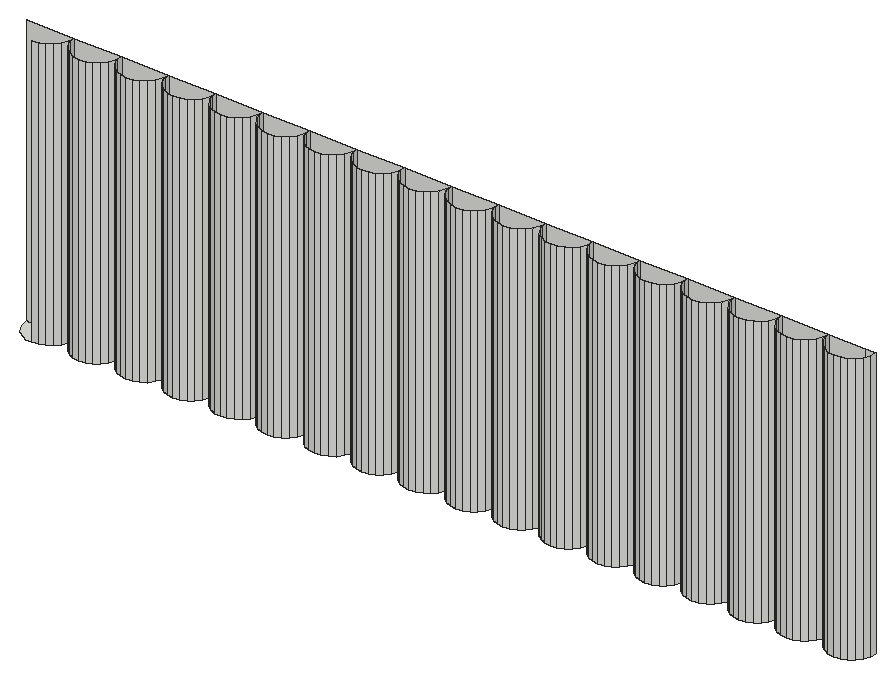
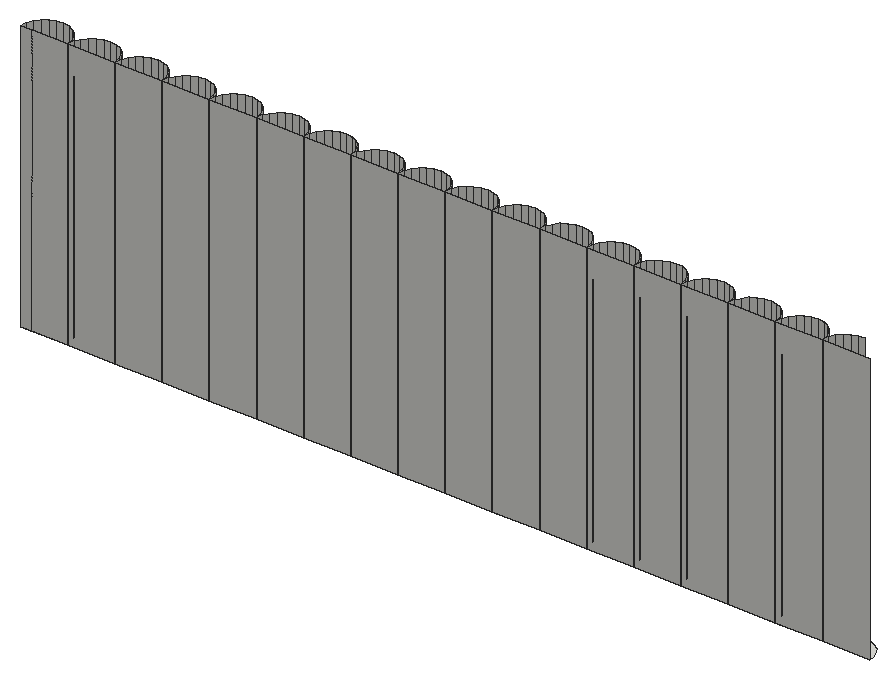
# SketchUp Ruby script. Lengths in inches.
U = 1.inch
M = Sketchup.active_model
def pt(a) = Geom::Point3d.new(a.map { |v| v * U })
def face(e, loops, mat)
  f = e.add_face(loops[0].map { |a| pt(a) })
  loops[1..].each { |l| e.add_face(l.map { |a| pt(a) }).erase! }
  f.material = f.back_material = mat if mat
  f
end
# faces: each face lists its corners as indices into pts; further lists are holes
def faces(e, pts, list, mat = nil) = list.each { |f| face(e, (f[0].is_a?(Array) ? f : [f]).map { |l| l.map { |i| pts[i] } }, mat) }
# xy, xz, yz: faces in a plane at the given z, y or x. An outline is a flat list of corners, or four numbers for a rectangle; further outlines are holes
def ring(l) = l.size == 4 ? [[l[0], l[1]], [l[2], l[1]], [l[2], l[3]], [l[0], l[3]]] : l.each_slice(2).to_a
def flat(e, list, mat, &to3) = list.each { |f| face(e, (f[0].is_a?(Array) ? f : [f]).map { |l| ring(l).map { |u, v| to3.(u, v) } }, mat) }
def xy(e, z, list, mat = nil) = flat(e, list, mat) { |x, y| [x, y, z] }
def xz(e, y, list, mat = nil) = flat(e, list, mat) { |x, z| [x, y, z] }
def yz(e, x, list, mat = nil) = flat(e, list, mat) { |y, z| [x, y, z] }
def lines(e, pts, list) = list.each { |a, b| e.add_line(pt(pts[a]), pt(pts[b])) }
# prism: a flat outline (further loops are holes) pulled along v
def prism(e, loops, v, mat = nil)
  f = face(e, loops, mat); d = Geom::Vector3d.new(v.map { |x| x * U })
  f.pushpull(f.normal.samedirection?(d) ? d.length : -d.length)
end
def box(e, o, s, mat = nil) = prism(e, [[o, [o[0] + s[0], o[1], o[2]], [o[0] + s[0], o[1] + s[1], o[2]], [o[0], o[1] + s[1], o[2]]]], [0, 0, s[2]], mat)
def at(x, y, z, deg = 0) = Geom::Transformation.translation(pt([x, y, z])) * Geom::Transformation.rotation(ORIGIN, Z_AXIS, deg.degrees)
def axes(o, x, y, z) = Geom::Transformation.new([*x, 0, *y, 0, *z, 0, *pt(o).to_a, 1])
def part(name) = M.definitions.add(name)
# library, detail: a bought-in or finely detailed component or shape, given as its bounding box
def library(name, o, s) = part(name).tap { |d| box(d.entities, o, s) }
def detail(e, o, s) = box(e.add_group.entities, o, s)
def put(e, d, t, mat = nil) = e.add_instance(d, t).tap { |i| i.material = mat if mat }
def group(e, t, mat = nil) = e.add_group.tap { |g| g.transformation = t; g.material = mat if mat }.entities
root = M.entities
xy(root,33.18,[[96.53,140.54,96.36,140.5625,96.2,140.63,96.0625,140.73,95.96,140.87,95.89,141.03,95.87,141.2,97.18,141.2,97.16,141.03,97.1,140.87,96.99,140.73,96.86,140.63,96.7,140.5625],[97.84,140.54,97.67,140.5625,97.51,140.63,97.375,140.73,97.27,140.87,97.21,141.03,97.18,141.2,98.5,141.2,98.47,141.03,98.41,140.87,98.3,140.73,98.17,140.63,98.01,140.5625],[99.15,140.54,98.98,140.5625,98.82,140.63,98.6875,140.73,98.58,140.87,98.52,141.03,98.5,141.2,99.81,141.2,99.79,141.03,99.72,140.87,99.62,140.73,99.48,140.63,99.32,140.5625],[100.46,140.54,100.3,140.5625,100.14,140.63,100,140.73,99.9,140.87,99.83,141.03,99.81,141.2,101.12,141.2,101.1,141.03,101.03,140.87,100.93,140.73,100.79,140.63,100.63,140.5625],[101.78,140.54,101.61,140.5625,101.45,140.63,101.3125,140.73,101.21,140.87,101.14,141.03,101.12,141.2,102.43,141.2,102.41,141.03,102.35,140.87,102.24,140.73,102.11,140.63,101.95,140.5625],
  [103.09,140.54,102.92,140.5625,102.76,140.63,102.625,140.73,102.52,140.87,102.46,141.03,102.43,141.2,103.75,141.2,103.72,141.03,103.66,140.87,103.55,140.73,103.42,140.63,103.26,140.5625],[104.4,140.54,104.23,140.5625,104.07,140.63,103.9375,140.73,103.83,140.87,103.77,141.03,103.75,141.2,105.06,141.2,105.04,141.03,104.97,140.87,104.87,140.73,104.73,140.63,104.57,140.5625],[105.71,140.54,105.55,140.5625,105.39,140.63,105.25,140.73,105.15,140.87,105.08,141.03,105.06,141.2,106.37,141.2,106.35,141.03,106.28,140.87,106.18,140.73,106.04,140.63,105.88,140.5625],[107.03,140.54,106.86,140.5625,106.7,140.63,106.5625,140.73,106.46,140.87,106.39,141.03,106.37,141.2,107.68,141.2,107.66,141.03,107.6,140.87,107.49,140.73,107.36,140.63,107.2,140.5625],[108.34,140.54,108.17,140.5625,108.01,140.63,107.875,140.73,107.77,140.87,107.71,141.03,107.68,141.2,109,141.2,108.97,141.03,108.91,140.87,108.8,140.73,108.67,140.63,108.51,140.5625],
  [109.65,140.54,109.48,140.5625,109.32,140.63,109.1875,140.73,109.08,140.87,109.02,141.03,109,141.2,110.31,141.2,110.29,141.03,110.22,140.87,110.12,140.73,109.98,140.63,109.82,140.5625],[110.96,140.54,110.8,140.5625,110.64,140.63,110.5,140.73,110.4,140.87,110.33,141.03,110.31,141.2,111.62,141.2,111.6,141.03,111.53,140.87,111.43,140.73,111.29,140.63,111.13,140.5625],[112.28,140.54,112.11,140.5625,111.95,140.63,111.8125,140.73,111.71,140.87,111.64,141.03,111.62,141.2,112.93,141.2,112.91,141.03,112.85,140.87,112.74,140.73,112.61,140.63,112.45,140.5625],[113.59,140.54,113.42,140.5625,113.26,140.63,113.125,140.73,113.02,140.87,112.96,141.03,112.93,141.2,114.25,141.2,114.22,141.03,114.16,140.87,114.05,140.73,113.92,140.63,113.76,140.5625],[114.9,140.54,114.73,140.5625,114.57,140.63,114.4375,140.73,114.33,140.87,114.27,141.03,114.25,141.2,115.56,141.2,115.54,141.03,115.47,140.87,115.37,140.73,115.23,140.63,115.07,140.5625],
  [116.21,140.54,116.05,140.5625,115.89,140.63,115.75,140.73,115.65,140.87,115.58,141.03,115.56,141.2,116.87,141.2,116.85,141.03,116.78,140.87,116.68,140.73,116.54,140.63,116.38,140.5625],[117.53,140.54,117.36,140.5625,117.2,140.63,117.0625,140.73,116.96,140.87,116.89,141.03,116.87,141.2,118.18,141.2,118.16,141.03,118.1,140.87,117.99,140.73,117.86,140.63,117.7,140.5625],[118.84,140.54,118.67,140.5625,118.51,140.63,118.375,140.73,118.27,140.87,118.21,141.03,118.18,141.2,119.5,141.2,119.47,141.03,119.41,140.87,119.3,140.73,119.17,140.63,119.01,140.5625]])
xz(root,141.2,[[95.87,33.18,97.18,40.6875],[97.18,33.18,98.5,40.6875],[98.5,33.18,99.81,40.6875],[99.81,33.18,101.12,40.6875],[101.12,33.18,102.43,40.6875],
  [102.43,33.18,103.75,40.6875],[103.75,33.18,105.06,40.6875],[105.06,33.18,106.37,40.6875],[106.37,33.18,107.68,40.6875],[107.68,33.18,109,40.6875],
  [109,33.18,110.31,40.6875],[110.31,33.18,111.62,40.6875],[111.62,33.18,112.93,40.6875],[112.93,33.18,114.25,40.6875],[114.25,33.18,115.56,40.6875],
  [115.56,33.18,116.87,40.6875],[116.87,33.18,118.18,40.6875],[118.18,33.18,119.1875,40.6875],[119.1875,33.18,119.5,40.6875]])
p = [[96.53,140.54,33.18],[96.7,140.5625,33.18],[96.7,140.5625,40.6875],[96.53,140.54,40.6875],[97.67,140.5625,33.18],[97.84,140.54,33.18],
  [97.84,140.54,40.6875],[97.67,140.5625,40.6875],[98.01,140.5625,33.18],[98.01,140.5625,40.6875],[98.98,140.5625,33.18],[99.15,140.54,33.18],
  [99.15,140.54,40.6875],[98.98,140.5625,40.6875],[99.32,140.5625,33.18],[99.32,140.5625,40.6875],[100.3,140.5625,33.18],[100.46,140.54,33.18],
  [100.46,140.54,40.6875],[100.3,140.5625,40.6875],[100.63,140.5625,33.18],[100.63,140.5625,40.6875],[101.61,140.5625,33.18],[101.78,140.54,33.18],
  [101.78,140.54,40.6875],[101.61,140.5625,40.6875],[101.95,140.5625,33.18],[101.95,140.5625,40.6875],[102.92,140.5625,33.18],[103.09,140.54,33.18],
  [103.09,140.54,40.6875],[102.92,140.5625,40.6875],[103.26,140.5625,33.18],[103.26,140.5625,40.6875],[104.23,140.5625,33.18],[104.4,140.54,33.18],
  [104.4,140.54,40.6875],[104.23,140.5625,40.6875],[104.57,140.5625,33.18],[104.57,140.5625,40.6875],[105.55,140.5625,33.18],[105.71,140.54,33.18],
  [105.71,140.54,40.6875],[105.55,140.5625,40.6875],[105.88,140.5625,33.18],[105.88,140.5625,40.6875],[106.86,140.5625,33.18],[107.03,140.54,33.18],
  [107.03,140.54,40.6875],[106.86,140.5625,40.6875],[107.2,140.5625,33.18],[107.2,140.5625,40.6875],[108.17,140.5625,33.18],[108.34,140.54,33.18],
  [108.34,140.54,40.6875],[108.17,140.5625,40.6875],[108.51,140.5625,33.18],[108.51,140.5625,40.6875],[109.48,140.5625,33.18],[109.65,140.54,33.18],
  [109.65,140.54,40.6875],[109.48,140.5625,40.6875],[109.82,140.5625,33.18],[109.82,140.5625,40.6875],[110.8,140.5625,33.18],[110.96,140.54,33.18],
  [110.96,140.54,40.6875],[110.8,140.5625,40.6875],[111.13,140.5625,33.18],[111.13,140.5625,40.6875],[112.11,140.5625,33.18],[112.28,140.54,33.18],
  [112.28,140.54,40.6875],[112.11,140.5625,40.6875],[112.45,140.5625,33.18],[112.45,140.5625,40.6875],[113.42,140.5625,33.18],[113.59,140.54,33.18],
  [113.59,140.54,40.6875],[113.42,140.5625,40.6875],[113.76,140.5625,33.18],[113.76,140.5625,40.6875],[114.73,140.5625,33.18],[114.9,140.54,33.18],
  [114.9,140.54,40.6875],[114.73,140.5625,40.6875],[115.07,140.5625,33.18],[115.07,140.5625,40.6875],[116.05,140.5625,33.18],[116.21,140.54,33.18],
  [116.21,140.54,40.6875],[116.05,140.5625,40.6875],[116.38,140.5625,33.18],[116.38,140.5625,40.6875],[117.36,140.5625,33.18],[117.53,140.54,33.18],
  [117.53,140.54,40.6875],[117.36,140.5625,40.6875],[117.7,140.5625,33.18],[117.7,140.5625,40.6875],[118.67,140.5625,33.18],[118.84,140.54,33.18],
  [118.84,140.54,40.6875],[118.67,140.5625,40.6875],[119.01,140.5625,33.18],[119.01,140.5625,40.6875],[96.86,140.63,33.18],[96.86,140.63,40.6875],
  [96.99,140.73,33.18],[96.99,140.73,40.6875],[97.375,140.73,33.18],[97.51,140.63,33.18],[97.51,140.63,40.6875],[97.375,140.73,40.6875],
  [98.17,140.63,33.18],[98.17,140.63,40.6875],[98.3,140.73,33.18],[98.3,140.73,40.6875],[98.6875,140.73,33.18],[98.82,140.63,33.18],
  [98.82,140.63,40.6875],[98.6875,140.73,40.6875],[99.48,140.63,33.18],[99.48,140.63,40.6875],[99.62,140.73,33.18],[99.62,140.73,40.6875],
  [100,140.73,33.18],[100.14,140.63,33.18],[100.14,140.63,40.6875],[100,140.73,40.6875],[100.79,140.63,33.18],[100.79,140.63,40.6875],
  [100.93,140.73,33.18],[100.93,140.73,40.6875],[101.3125,140.73,33.18],[101.45,140.63,33.18],[101.45,140.63,40.6875],[101.3125,140.73,40.6875],
  [102.11,140.63,33.18],[102.11,140.63,40.6875],[102.24,140.73,33.18],[102.24,140.73,40.6875],[102.625,140.73,33.18],[102.76,140.63,33.18],
  [102.76,140.63,40.6875],[102.625,140.73,40.6875],[103.42,140.63,33.18],[103.42,140.63,40.6875],[103.55,140.73,33.18],[103.55,140.73,40.6875],
  [103.9375,140.73,33.18],[104.07,140.63,33.18],[104.07,140.63,40.6875],[103.9375,140.73,40.6875],[104.73,140.63,33.18],[104.73,140.63,40.6875],
  [104.87,140.73,33.18],[104.87,140.73,40.6875],[105.25,140.73,33.18],[105.39,140.63,33.18],[105.39,140.63,40.6875],[105.25,140.73,40.6875],
  [106.04,140.63,33.18],[106.04,140.63,40.6875],[106.18,140.73,33.18],[106.18,140.73,40.6875],[106.5625,140.73,33.18],[106.7,140.63,33.18],
  [106.7,140.63,40.6875],[106.5625,140.73,40.6875],[107.36,140.63,33.18],[107.36,140.63,40.6875],[107.49,140.73,33.18],[107.49,140.73,40.6875],
  [107.875,140.73,33.18],[108.01,140.63,33.18],[108.01,140.63,40.6875],[107.875,140.73,40.6875],[108.67,140.63,33.18],[108.67,140.63,40.6875],
  [108.8,140.73,33.18],[108.8,140.73,40.6875],[109.1875,140.73,33.18],[109.32,140.63,33.18],[109.32,140.63,40.6875],[109.1875,140.73,40.6875],
  [109.98,140.63,33.18],[109.98,140.63,40.6875],[110.12,140.73,33.18],[110.12,140.73,40.6875],[110.5,140.73,33.18],[110.64,140.63,33.18],
  [110.64,140.63,40.6875],[110.5,140.73,40.6875],[111.29,140.63,33.18],[111.29,140.63,40.6875],[111.43,140.73,33.18],[111.43,140.73,40.6875],
  [111.8125,140.73,33.18],[111.95,140.63,33.18],[111.95,140.63,40.6875],[111.8125,140.73,40.6875],[112.61,140.63,33.18],[112.61,140.63,40.6875],
  [112.74,140.73,33.18],[112.74,140.73,40.6875],[113.125,140.73,33.18],[113.26,140.63,33.18],[113.26,140.63,40.6875],[113.125,140.73,40.6875],
  [113.92,140.63,33.18],[113.92,140.63,40.6875],[114.05,140.73,33.18],[114.05,140.73,40.6875],[114.4375,140.73,33.18],[114.57,140.63,33.18],
  [114.57,140.63,40.6875],[114.4375,140.73,40.6875],[115.23,140.63,33.18],[115.23,140.63,40.6875],[115.37,140.73,33.18],[115.37,140.73,40.6875],
  [115.75,140.73,33.18],[115.89,140.63,33.18],[115.89,140.63,40.6875],[115.75,140.73,40.6875],[116.54,140.63,33.18],[116.54,140.63,40.6875],
  [116.68,140.73,33.18],[116.68,140.73,40.6875],[117.0625,140.73,33.18],[117.2,140.63,33.18],[117.2,140.63,40.6875],[117.0625,140.73,40.6875],
  [117.86,140.63,33.18],[117.86,140.63,40.6875],[117.99,140.73,33.18],[117.99,140.73,40.6875],[118.375,140.73,33.18],[118.51,140.63,33.18],
  [118.51,140.63,40.6875],[118.375,140.73,40.6875],[119.17,140.63,33.18],[119.17,140.63,40.6875],[119.3,140.73,33.18],[119.3,140.73,40.6875],
  [119.1875,140.64,40.6875],[97.1,140.87,33.18],[97.1,140.87,40.6875],[97.27,140.87,33.18],[97.27,140.87,40.6875],[98.41,140.87,33.18],
  [98.41,140.87,40.6875],[98.58,140.87,33.18],[98.58,140.87,40.6875],[99.72,140.87,33.18],[99.72,140.87,40.6875],[99.9,140.87,33.18],
  [99.9,140.87,40.6875],[101.03,140.87,33.18],[101.03,140.87,40.6875],[101.21,140.87,33.18],[101.21,140.87,40.6875],[102.35,140.87,33.18],
  [102.35,140.87,40.6875],[102.52,140.87,33.18],[102.52,140.87,40.6875],[103.66,140.87,33.18],[103.66,140.87,40.6875],[103.83,140.87,33.18],
  [103.83,140.87,40.6875],[104.97,140.87,33.18],[104.97,140.87,40.6875],[105.15,140.87,33.18],[105.15,140.87,40.6875],[106.28,140.87,33.18],
  [106.28,140.87,40.6875],[106.46,140.87,33.18],[106.46,140.87,40.6875],[107.6,140.87,33.18],[107.6,140.87,40.6875],[107.77,140.87,33.18],
  [107.77,140.87,40.6875],[108.91,140.87,33.18],[108.91,140.87,40.6875],[109.08,140.87,33.18],[109.08,140.87,40.6875],[110.22,140.87,33.18],
  [110.22,140.87,40.6875],[110.4,140.87,33.18],[110.4,140.87,40.6875],[111.53,140.87,33.18],[111.53,140.87,40.6875],[111.71,140.87,33.18],
  [111.71,140.87,40.6875],[112.85,140.87,33.18],[112.85,140.87,40.6875],[113.02,140.87,33.18],[113.02,140.87,40.6875],[114.16,140.87,33.18],
  [114.16,140.87,40.6875],[114.33,140.87,33.18],[114.33,140.87,40.6875],[115.47,140.87,33.18],[115.47,140.87,40.6875],[115.65,140.87,33.18],
  [115.65,140.87,40.6875],[116.78,140.87,33.18],[116.78,140.87,40.6875],[116.96,140.87,33.18],[116.96,140.87,40.6875],[118.1,140.87,33.18],
  [118.1,140.87,40.6875],[118.27,140.87,33.18],[118.27,140.87,40.6875],[119.41,140.87,33.18],[119.41,140.87,40.6875],[97.16,141.03,33.18],
  [97.16,141.03,40.6875],[97.21,141.03,33.18],[97.21,141.03,40.6875],[98.47,141.03,33.18],[98.47,141.03,40.6875],[98.52,141.03,33.18],
  [98.52,141.03,40.6875],[99.79,141.03,33.18],[99.79,141.03,40.6875],[99.83,141.03,33.18],[99.83,141.03,40.6875],[101.1,141.03,33.18],
  [101.1,141.03,40.6875],[101.14,141.03,33.18],[101.14,141.03,40.6875],[102.41,141.03,33.18],[102.41,141.03,40.6875],[102.46,141.03,33.18],
  [102.46,141.03,40.6875],[103.72,141.03,33.18],[103.72,141.03,40.6875],[103.77,141.03,33.18],[103.77,141.03,40.6875],[105.04,141.03,33.18],
  [105.04,141.03,40.6875],[105.08,141.03,33.18],[105.08,141.03,40.6875],[106.35,141.03,33.18],[106.35,141.03,40.6875],[106.39,141.03,33.18],
  [106.39,141.03,40.6875],[107.66,141.03,33.18],[107.66,141.03,40.6875],[107.71,141.03,33.18],[107.71,141.03,40.6875],[108.97,141.03,33.18],
  [108.97,141.03,40.6875],[109.02,141.03,33.18],[109.02,141.03,40.6875],[110.29,141.03,33.18],[110.29,141.03,40.6875],[110.33,141.03,33.18],
  [110.33,141.03,40.6875],[111.6,141.03,33.18],[111.6,141.03,40.6875],[111.64,141.03,33.18],[111.64,141.03,40.6875],[112.91,141.03,33.18],
  [112.91,141.03,40.6875],[112.96,141.03,33.18],[112.96,141.03,40.6875],[114.22,141.03,33.18],[114.22,141.03,40.6875],[114.27,141.03,33.18],
  [114.27,141.03,40.6875],[115.54,141.03,33.18],[115.54,141.03,40.6875],[115.58,141.03,33.18],[115.58,141.03,40.6875],[116.85,141.03,33.18],
  [116.85,141.03,40.6875],[116.89,141.03,33.18],[116.89,141.03,40.6875],[118.16,141.03,33.18],[118.16,141.03,40.6875],[118.21,141.03,33.18],
  [118.21,141.03,40.6875],[119.47,141.03,33.18],[119.47,141.03,40.6875],[97.18,141.2,33.18],[97.18,141.2,40.6875],[98.5,141.2,33.18],
  [98.5,141.2,40.6875],[99.81,141.2,33.18],[99.81,141.2,40.6875],[101.12,141.2,33.18],[101.12,141.2,40.6875],[102.43,141.2,33.18],
  [102.43,141.2,40.6875],[103.75,141.2,33.18],[103.75,141.2,40.6875],[105.06,141.2,33.18],[105.06,141.2,40.6875],[106.37,141.2,33.18],
  [106.37,141.2,40.6875],[107.68,141.2,33.18],[107.68,141.2,40.6875],[109,141.2,33.18],[109,141.2,40.6875],[110.31,141.2,33.18],
  [110.31,141.2,40.6875],[111.62,141.2,33.18],[111.62,141.2,40.6875],[112.93,141.2,33.18],[112.93,141.2,40.6875],[114.25,141.2,33.18],
  [114.25,141.2,40.6875],[115.56,141.2,33.18],[115.56,141.2,40.6875],[116.87,141.2,33.18],[116.87,141.2,40.6875],[118.18,141.2,33.18],
  [118.18,141.2,40.6875],[119.5,141.2,33.18],[119.5,141.2,40.6875]]
faces(root,p,[[0,1,2,3],[4,5,6,7],[5,8,9,6],[10,11,12,13],[11,14,15,12],[16,17,18,19],[17,20,21,18],[22,23,24,25],
  [23,26,27,24],[28,29,30,31],[29,32,33,30],[34,35,36,37],[35,38,39,36],[40,41,42,43],[41,44,45,42],[46,47,48,49],
  [47,50,51,48],[52,53,54,55],[53,56,57,54],[58,59,60,61],[59,62,63,60],[64,65,66,67],[65,68,69,66],[70,71,72,73],
  [71,74,75,72],[76,77,78,79],[77,80,81,78],[82,83,84,85],[83,86,87,84],[88,89,90,91],[89,92,93,90],[94,95,96,97],
  [95,98,99,96],[100,101,102,103],[101,104,105,102],[1,106,107,2],[106,108,109,107],[110,111,112,113],[111,4,7,112],[8,114,115,9],
  [114,116,117,115],[118,119,120,121],[119,10,13,120],[14,122,123,15],[122,124,125,123],[126,127,128,129],[127,16,19,128],[20,130,131,21],
  [130,132,133,131],[134,135,136,137],[135,22,25,136],[26,138,139,27],[138,140,141,139],[142,143,144,145],[143,28,31,144],[32,146,147,33],
  [146,148,149,147],[150,151,152,153],[151,34,37,152],[38,154,155,39],[154,156,157,155],[158,159,160,161],[159,40,43,160],[44,162,163,45],
  [162,164,165,163],[166,167,168,169],[167,46,49,168],[50,170,171,51],[170,172,173,171],[174,175,176,177],[175,52,55,176],[56,178,179,57],
  [178,180,181,179],[182,183,184,185],[183,58,61,184],[62,186,187,63],[186,188,189,187],[190,191,192,193],[191,64,67,192],[68,194,195,69],
  [194,196,197,195],[198,199,200,201],[199,70,73,200],[74,202,203,75],[202,204,205,203],[206,207,208,209],[207,76,79,208],[80,210,211,81],
  [210,212,213,211],[214,215,216,217],[215,82,85,216],[86,218,219,87],[218,220,221,219],[222,223,224,225],[223,88,91,224],[92,226,227,93],
  [226,228,229,227],[230,231,232,233],[231,94,97,232],[98,234,235,99],[234,236,237,235],[238,239,240,241],[239,100,103,240],[104,242,243,105],
  [242,244,245,246,243],[108,247,248,109],[249,110,113,250],[116,251,252,117],[253,118,121,254],[124,255,256,125],[257,126,129,258],[132,259,260,133],
  [261,134,137,262],[140,263,264,141],[265,142,145,266],[148,267,268,149],[269,150,153,270],[156,271,272,157],[273,158,161,274],[164,275,276,165],
  [277,166,169,278],[172,279,280,173],[281,174,177,282],[180,283,284,181],[285,182,185,286],[188,287,288,189],[289,190,193,290],[196,291,292,197],
  [293,198,201,294],[204,295,296,205],[297,206,209,298],[212,299,300,213],[301,214,217,302],[220,303,304,221],[305,222,225,306],[228,307,308,229],
  [309,230,233,310],[236,311,312,237],[313,238,241,314],[244,315,316,245],[247,317,318,248],[319,249,250,320],[251,321,322,252],[323,253,254,324],
  [255,325,326,256],[327,257,258,328],[259,329,330,260],[331,261,262,332],[263,333,334,264],[335,265,266,336],[267,337,338,268],[339,269,270,340],
  [271,341,342,272],[343,273,274,344],[275,345,346,276],[347,277,278,348],[279,349,350,280],[351,281,282,352],[283,353,354,284],[355,285,286,356],
  [287,357,358,288],[359,289,290,360],[291,361,362,292],[363,293,294,364],[295,365,366,296],[367,297,298,368],[299,369,370,300],[371,301,302,372],
  [303,373,374,304],[375,305,306,376],[307,377,378,308],[379,309,310,380],[311,381,382,312],[383,313,314,384],[315,385,386,316],[317,387,388,318],
  [387,319,320,388],[321,389,390,322],[389,323,324,390],[325,391,392,326],[391,327,328,392],[329,393,394,330],[393,331,332,394],[333,395,396,334],
  [395,335,336,396],[337,397,398,338],[397,339,340,398],[341,399,400,342],[399,343,344,400],[345,401,402,346],[401,347,348,402],[349,403,404,350],
  [403,351,352,404],[353,405,406,354],[405,355,356,406],[357,407,408,358],[407,359,360,408],[361,409,410,362],[409,363,364,410],[365,411,412,366],
  [411,367,368,412],[369,413,414,370],[413,371,372,414],[373,415,416,374],[415,375,376,416],[377,417,418,378],[417,379,380,418],[381,419,420,382],
  [419,383,384,420],[385,421,422,386]])
